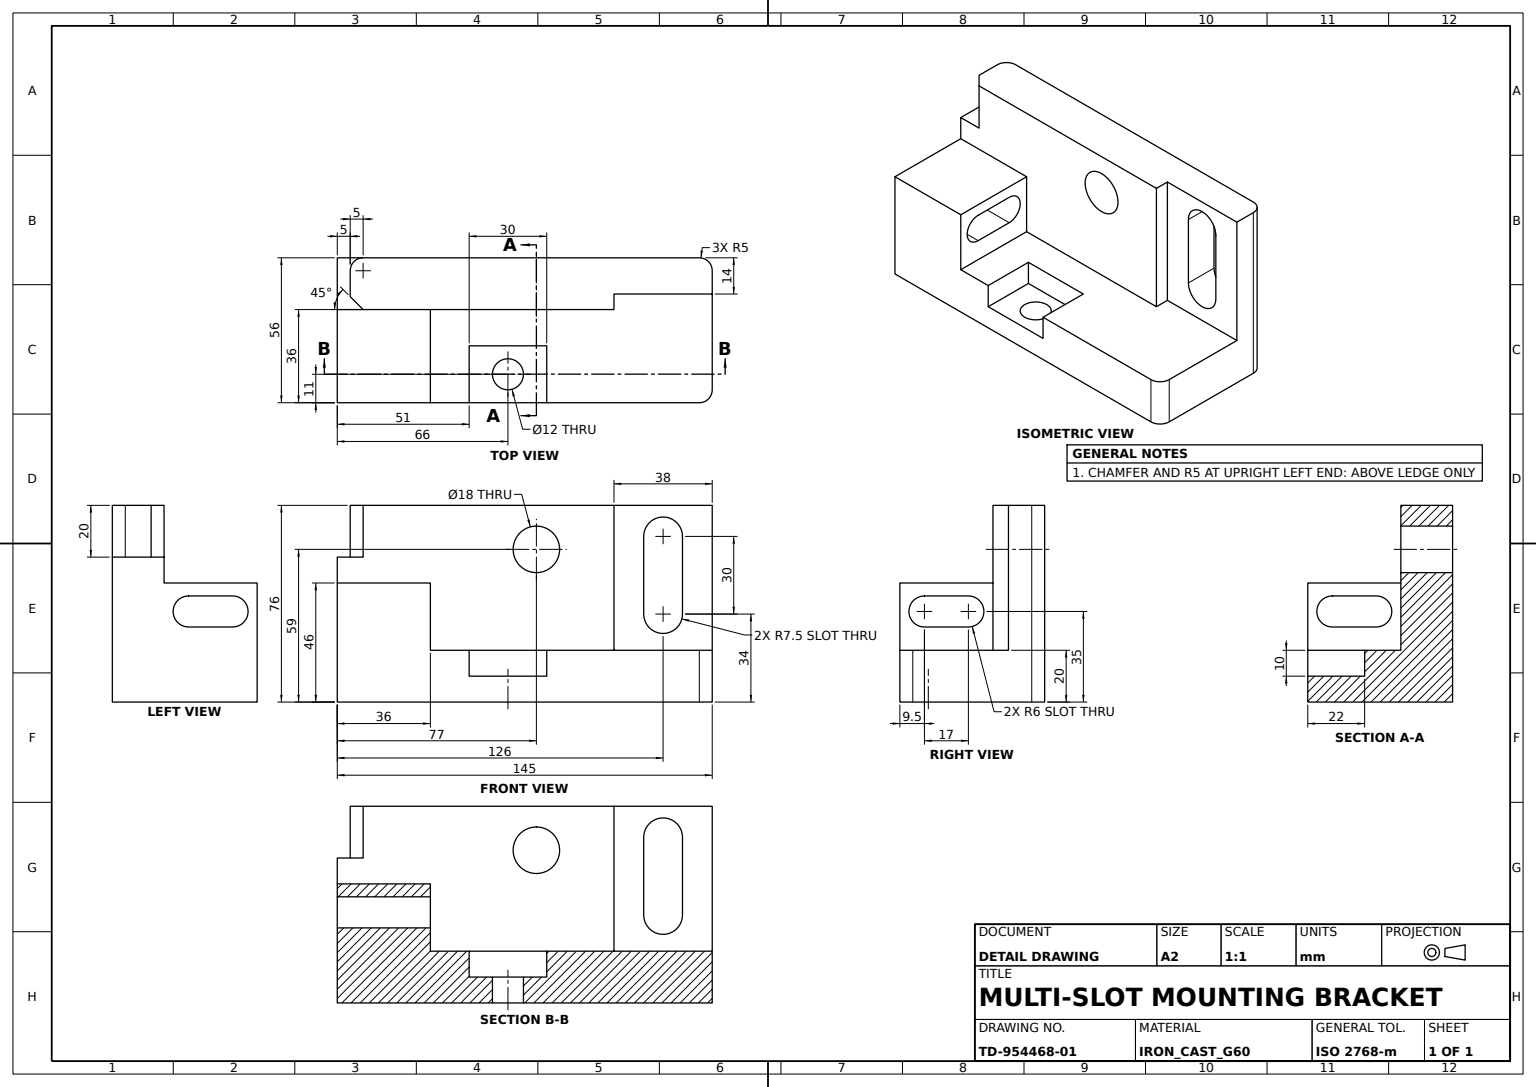
ISO-10303-21;
HEADER;
FILE_DESCRIPTION((''),'2;1');
FILE_NAME('','',(''),(''),'','','');
FILE_SCHEMA(('AUTOMOTIVE_DESIGN'));
ENDSEC;
DATA;
#1=APPLICATION_CONTEXT('');
#2=PRODUCT_CONTEXT('',#1,'mechanical');
#3=PRODUCT('','','',(#2));
#4=PRODUCT_DEFINITION_FORMATION('','',#3);
#5=PRODUCT_DEFINITION_CONTEXT('',#1,'design');
#6=PRODUCT_DEFINITION('','',#4,#5);
#7=PRODUCT_DEFINITION_SHAPE('','',#6);
#8=(LENGTH_UNIT()NAMED_UNIT(*)SI_UNIT(.MILLI.,.METRE.));
#9=(NAMED_UNIT(*)PLANE_ANGLE_UNIT()SI_UNIT($,.RADIAN.));
#10=(NAMED_UNIT(*)SI_UNIT($,.STERADIAN.)SOLID_ANGLE_UNIT());
#11=UNCERTAINTY_MEASURE_WITH_UNIT(LENGTH_MEASURE(0.005),#8,'distance_accuracy_value','');
#12=(GEOMETRIC_REPRESENTATION_CONTEXT(3)GLOBAL_UNCERTAINTY_ASSIGNED_CONTEXT((#11))GLOBAL_UNIT_ASSIGNED_CONTEXT((#8,#9,#10))REPRESENTATION_CONTEXT('',''));
#13=CARTESIAN_POINT('',(-12.5,-17.,10.));
#14=VERTEX_POINT('',#13);
#15=CARTESIAN_POINT('',(-6.5,-17.,10.));
#16=DIRECTION('',(0.,0.,-1.));
#17=DIRECTION('',(-1.,0.,0.));
#18=AXIS2_PLACEMENT_3D('',#15,#16,#17);
#19=CIRCLE('',#18,6.);
#20=EDGE_CURVE('',#14,#14,#19,.T.);
#21=ORIENTED_EDGE('',*,*,#20,.T.);
#22=EDGE_LOOP('',(#21));
#23=FACE_BOUND('',#22,.T.);
#24=CARTESIAN_POINT('',(-21.5,-6.,10.));
#25=VERTEX_POINT('',#24);
#26=CARTESIAN_POINT('',(-21.5,-28.,10.));
#27=VERTEX_POINT('',#26);
#28=CARTESIAN_POINT('',(-21.5,-40.,10.));
#29=DIRECTION('',(0.,1.,0.));
#30=VECTOR('',#29,1000.);
#31=LINE('',#28,#30);
#32=EDGE_CURVE('',#25,#27,#31,.F.);
#33=ORIENTED_EDGE('',*,*,#32,.T.);
#34=CARTESIAN_POINT('',(8.5,-28.,10.));
#35=VERTEX_POINT('',#34);
#36=CARTESIAN_POINT('',(72.5,-28.,10.));
#37=DIRECTION('',(1.,0.,0.));
#38=VECTOR('',#37,1000.);
#39=LINE('',#36,#38);
#40=EDGE_CURVE('',#27,#35,#39,.T.);
#41=ORIENTED_EDGE('',*,*,#40,.T.);
#42=CARTESIAN_POINT('',(8.5,-6.,10.));
#43=VERTEX_POINT('',#42);
#44=DIRECTION('',(0.,-1.,0.));
#45=VECTOR('',#44,1000.);
#46=LINE('',#42,#45);
#47=EDGE_CURVE('',#35,#43,#46,.F.);
#48=ORIENTED_EDGE('',*,*,#47,.T.);
#49=LINE('',#24,#38);
#50=EDGE_CURVE('',#43,#25,#49,.F.);
#51=ORIENTED_EDGE('',*,*,#50,.T.);
#52=EDGE_LOOP('',(#33,#41,#48,#51));
#53=FACE_BOUND('',#52,.T.);
#54=CARTESIAN_POINT('',(0.,0.,10.));
#55=AXIS2_PLACEMENT_3D('',#54,#16,#17);
#56=PLANE('',#55);
#57=ADVANCED_FACE('',(#23,#53),#56,.F.);
#58=CARTESIAN_POINT('',(-21.5,-28.,20.));
#59=VERTEX_POINT('',#58);
#60=CARTESIAN_POINT('',(-21.5,-6.,20.));
#61=VERTEX_POINT('',#60);
#62=CARTESIAN_POINT('',(-21.5,0.,20.));
#63=LINE('',#62,#30);
#64=EDGE_CURVE('',#59,#61,#63,.T.);
#65=ORIENTED_EDGE('',*,*,#64,.T.);
#66=CARTESIAN_POINT('',(8.5,-6.,20.));
#67=VERTEX_POINT('',#66);
#68=CARTESIAN_POINT('',(0.,-6.,20.));
#69=LINE('',#68,#38);
#70=EDGE_CURVE('',#61,#67,#69,.T.);
#71=ORIENTED_EDGE('',*,*,#70,.T.);
#72=CARTESIAN_POINT('',(8.5,-28.,20.));
#73=VERTEX_POINT('',#72);
#74=CARTESIAN_POINT('',(8.5,0.,20.));
#75=LINE('',#74,#45);
#76=EDGE_CURVE('',#67,#73,#75,.T.);
#77=ORIENTED_EDGE('',*,*,#76,.T.);
#78=CARTESIAN_POINT('',(67.5,-28.,20.));
#79=VERTEX_POINT('',#78);
#80=CARTESIAN_POINT('',(72.5,-28.,20.));
#81=VECTOR('',#17,1000.);
#82=LINE('',#80,#81);
#83=EDGE_CURVE('',#79,#73,#82,.T.);
#84=ORIENTED_EDGE('',*,*,#83,.F.);
#85=CARTESIAN_POINT('',(72.5,-23.,20.));
#86=VERTEX_POINT('',#85);
#87=CARTESIAN_POINT('',(67.5,-23.,20.));
#88=AXIS2_PLACEMENT_3D('',#87,#16,#17);
#89=CIRCLE('',#88,5.);
#90=EDGE_CURVE('',#79,#86,#89,.F.);
#91=ORIENTED_EDGE('',*,*,#90,.T.);
#92=CARTESIAN_POINT('',(72.5,14.,20.));
#93=VERTEX_POINT('',#92);
#94=CARTESIAN_POINT('',(72.5,28.,20.));
#95=LINE('',#94,#45);
#96=EDGE_CURVE('',#93,#86,#95,.T.);
#97=ORIENTED_EDGE('',*,*,#96,.F.);
#98=CARTESIAN_POINT('',(34.5,14.,20.));
#99=VERTEX_POINT('',#98);
#100=LINE('',#92,#81);
#101=EDGE_CURVE('',#99,#93,#100,.F.);
#102=ORIENTED_EDGE('',*,*,#101,.F.);
#103=CARTESIAN_POINT('',(34.5,8.,20.));
#104=VERTEX_POINT('',#103);
#105=LINE('',#98,#45);
#106=EDGE_CURVE('',#104,#99,#105,.F.);
#107=ORIENTED_EDGE('',*,*,#106,.F.);
#108=CARTESIAN_POINT('',(-36.5,8.,20.));
#109=VERTEX_POINT('',#108);
#110=CARTESIAN_POINT('',(0.,8.,20.));
#111=LINE('',#110,#81);
#112=EDGE_CURVE('',#104,#109,#111,.T.);
#113=ORIENTED_EDGE('',*,*,#112,.T.);
#114=CARTESIAN_POINT('',(-36.5,-28.,20.));
#115=VERTEX_POINT('',#114);
#116=CARTESIAN_POINT('',(-36.5,0.,20.));
#117=LINE('',#116,#45);
#118=EDGE_CURVE('',#109,#115,#117,.T.);
#119=ORIENTED_EDGE('',*,*,#118,.T.);
#120=EDGE_CURVE('',#59,#115,#82,.T.);
#121=ORIENTED_EDGE('',*,*,#120,.F.);
#122=EDGE_LOOP('',(#65,#71,#77,#84,#91,#97,#102,#107,#113,#119,#121));
#123=FACE_BOUND('',#122,.T.);
#124=CARTESIAN_POINT('',(0.,0.,20.));
#125=AXIS2_PLACEMENT_3D('',#124,#16,#17);
#126=PLANE('',#125);
#127=ADVANCED_FACE('',(#123),#126,.F.);
#128=CARTESIAN_POINT('',(-72.5,8.,56.));
#129=VERTEX_POINT('',#128);
#130=CARTESIAN_POINT('',(-62.5,8.,56.));
#131=VERTEX_POINT('',#130);
#132=CARTESIAN_POINT('',(72.5,8.,56.));
#133=LINE('',#132,#38);
#134=EDGE_CURVE('',#129,#131,#133,.T.);
#135=ORIENTED_EDGE('',*,*,#134,.T.);
#136=CARTESIAN_POINT('',(-67.5,13.,56.));
#137=VERTEX_POINT('',#136);
#138=CARTESIAN_POINT('',(-86.5,32.,56.));
#139=DIRECTION('',(-0.707106781,0.707106781,0.));
#140=VECTOR('',#139,1000.);
#141=LINE('',#138,#140);
#142=EDGE_CURVE('',#131,#137,#141,.T.);
#143=ORIENTED_EDGE('',*,*,#142,.T.);
#144=CARTESIAN_POINT('',(-67.5,23.,56.));
#145=VERTEX_POINT('',#144);
#146=CARTESIAN_POINT('',(-67.5,46.,56.));
#147=LINE('',#146,#45);
#148=EDGE_CURVE('',#137,#145,#147,.F.);
#149=ORIENTED_EDGE('',*,*,#148,.T.);
#150=CARTESIAN_POINT('',(-62.5,28.,56.));
#151=VERTEX_POINT('',#150);
#152=CARTESIAN_POINT('',(-62.5,23.,56.));
#153=AXIS2_PLACEMENT_3D('',#152,#16,#17);
#154=CIRCLE('',#153,5.);
#155=EDGE_CURVE('',#145,#151,#154,.T.);
#156=ORIENTED_EDGE('',*,*,#155,.T.);
#157=CARTESIAN_POINT('',(-72.5,28.,56.));
#158=VERTEX_POINT('',#157);
#159=LINE('',#157,#81);
#160=EDGE_CURVE('',#151,#158,#159,.T.);
#161=ORIENTED_EDGE('',*,*,#160,.T.);
#162=CARTESIAN_POINT('',(-72.5,46.,56.));
#163=LINE('',#162,#45);
#164=EDGE_CURVE('',#158,#129,#163,.T.);
#165=ORIENTED_EDGE('',*,*,#164,.T.);
#166=EDGE_LOOP('',(#135,#143,#149,#156,#161,#165));
#167=FACE_BOUND('',#166,.T.);
#168=AXIS2_PLACEMENT_3D('',#162,#16,#17);
#169=PLANE('',#168);
#170=ADVANCED_FACE('',(#167),#169,.F.);
#171=CARTESIAN_POINT('',(-72.5,8.,46.));
#172=VERTEX_POINT('',#171);
#173=CARTESIAN_POINT('',(-36.5,8.,46.));
#174=VERTEX_POINT('',#173);
#175=LINE('',#171,#38);
#176=EDGE_CURVE('',#172,#174,#175,.T.);
#177=ORIENTED_EDGE('',*,*,#176,.F.);
#178=CARTESIAN_POINT('',(-72.5,-28.,46.));
#179=VERTEX_POINT('',#178);
#180=LINE('',#178,#30);
#181=EDGE_CURVE('',#179,#172,#180,.T.);
#182=ORIENTED_EDGE('',*,*,#181,.F.);
#183=CARTESIAN_POINT('',(-36.5,-28.,46.));
#184=VERTEX_POINT('',#183);
#185=LINE('',#183,#81);
#186=EDGE_CURVE('',#184,#179,#185,.T.);
#187=ORIENTED_EDGE('',*,*,#186,.F.);
#188=LINE('',#173,#45);
#189=EDGE_CURVE('',#174,#184,#188,.T.);
#190=ORIENTED_EDGE('',*,*,#189,.F.);
#191=EDGE_LOOP('',(#177,#182,#187,#190));
#192=FACE_BOUND('',#191,.T.);
#193=CARTESIAN_POINT('',(0.,0.,46.));
#194=AXIS2_PLACEMENT_3D('',#193,#16,#17);
#195=PLANE('',#194);
#196=ADVANCED_FACE('',(#192),#195,.F.);
#197=CARTESIAN_POINT('',(46.,14.,34.));
#198=VERTEX_POINT('',#197);
#199=CARTESIAN_POINT('',(46.,14.,64.));
#200=VERTEX_POINT('',#199);
#201=CARTESIAN_POINT('',(46.,14.,87.5));
#202=DIRECTION('',(0.,0.,1.));
#203=VECTOR('',#202,1000.);
#204=LINE('',#201,#203);
#205=EDGE_CURVE('',#198,#200,#204,.T.);
#206=ORIENTED_EDGE('',*,*,#205,.T.);
#207=CARTESIAN_POINT('',(61.,14.,64.));
#208=VERTEX_POINT('',#207);
#209=CARTESIAN_POINT('',(53.5,14.,64.));
#210=AXIS2_PLACEMENT_3D('',#209,#44,#37);
#211=CIRCLE('',#210,7.5);
#212=EDGE_CURVE('',#200,#208,#211,.F.);
#213=ORIENTED_EDGE('',*,*,#212,.T.);
#214=CARTESIAN_POINT('',(61.,14.,34.));
#215=VERTEX_POINT('',#214);
#216=CARTESIAN_POINT('',(61.,14.,87.5));
#217=VECTOR('',#16,1000.);
#218=LINE('',#216,#217);
#219=EDGE_CURVE('',#208,#215,#218,.T.);
#220=ORIENTED_EDGE('',*,*,#219,.T.);
#221=CARTESIAN_POINT('',(53.5,14.,34.));
#222=AXIS2_PLACEMENT_3D('',#221,#44,#37);
#223=CIRCLE('',#222,7.5);
#224=EDGE_CURVE('',#215,#198,#223,.F.);
#225=ORIENTED_EDGE('',*,*,#224,.T.);
#226=EDGE_LOOP('',(#206,#213,#220,#225));
#227=FACE_BOUND('',#226,.T.);
#228=ORIENTED_EDGE('',*,*,#101,.T.);
#229=CARTESIAN_POINT('',(72.5,14.,76.));
#230=VERTEX_POINT('',#229);
#231=CARTESIAN_POINT('',(72.5,14.,87.5));
#232=LINE('',#231,#217);
#233=EDGE_CURVE('',#93,#230,#232,.F.);
#234=ORIENTED_EDGE('',*,*,#233,.T.);
#235=CARTESIAN_POINT('',(34.5,14.,76.));
#236=VERTEX_POINT('',#235);
#237=LINE('',#229,#38);
#238=EDGE_CURVE('',#236,#230,#237,.T.);
#239=ORIENTED_EDGE('',*,*,#238,.F.);
#240=CARTESIAN_POINT('',(34.5,14.,87.5));
#241=LINE('',#240,#217);
#242=EDGE_CURVE('',#236,#99,#241,.T.);
#243=ORIENTED_EDGE('',*,*,#242,.T.);
#244=EDGE_LOOP('',(#228,#234,#239,#243));
#245=FACE_BOUND('',#244,.T.);
#246=AXIS2_PLACEMENT_3D('',#231,#44,#37);
#247=PLANE('',#246);
#248=ADVANCED_FACE('',(#227,#245),#247,.T.);
#249=ORIENTED_EDGE('',*,*,#212,.F.);
#250=CARTESIAN_POINT('',(46.,28.,64.));
#251=VERTEX_POINT('',#250);
#252=CARTESIAN_POINT('',(46.,76.5,64.));
#253=LINE('',#252,#45);
#254=EDGE_CURVE('',#200,#251,#253,.F.);
#255=ORIENTED_EDGE('',*,*,#254,.T.);
#256=CARTESIAN_POINT('',(61.,28.,64.));
#257=VERTEX_POINT('',#256);
#258=CARTESIAN_POINT('',(53.5,28.,64.));
#259=AXIS2_PLACEMENT_3D('',#258,#29,#202);
#260=CIRCLE('',#259,7.5);
#261=EDGE_CURVE('',#257,#251,#260,.F.);
#262=ORIENTED_EDGE('',*,*,#261,.F.);
#263=CARTESIAN_POINT('',(61.,76.5,64.));
#264=LINE('',#263,#45);
#265=EDGE_CURVE('',#208,#257,#264,.F.);
#266=ORIENTED_EDGE('',*,*,#265,.F.);
#267=EDGE_LOOP('',(#249,#255,#262,#266));
#268=FACE_BOUND('',#267,.T.);
#269=CARTESIAN_POINT('',(53.5,76.5,64.));
#270=AXIS2_PLACEMENT_3D('',#269,#44,#16);
#271=CYLINDRICAL_SURFACE('',#270,7.5);
#272=ADVANCED_FACE('',(#268),#271,.F.);
#273=CARTESIAN_POINT('',(67.5,28.,76.));
#274=VERTEX_POINT('',#273);
#275=CARTESIAN_POINT('',(-62.5,28.,76.));
#276=VERTEX_POINT('',#275);
#277=CARTESIAN_POINT('',(72.5,28.,76.));
#278=LINE('',#277,#81);
#279=EDGE_CURVE('',#274,#276,#278,.T.);
#280=ORIENTED_EDGE('',*,*,#279,.T.);
#281=CARTESIAN_POINT('',(-67.5,23.,76.));
#282=VERTEX_POINT('',#281);
#283=CARTESIAN_POINT('',(-62.5,23.,76.));
#284=AXIS2_PLACEMENT_3D('',#283,#202,#37);
#285=CIRCLE('',#284,5.);
#286=EDGE_CURVE('',#276,#282,#285,.T.);
#287=ORIENTED_EDGE('',*,*,#286,.T.);
#288=CARTESIAN_POINT('',(-67.5,13.,76.));
#289=VERTEX_POINT('',#288);
#290=CARTESIAN_POINT('',(-67.5,8.,76.));
#291=LINE('',#290,#30);
#292=EDGE_CURVE('',#289,#282,#291,.T.);
#293=ORIENTED_EDGE('',*,*,#292,.F.);
#294=CARTESIAN_POINT('',(-62.5,8.,76.));
#295=VERTEX_POINT('',#294);
#296=CARTESIAN_POINT('',(5.,-59.5,76.));
#297=DIRECTION('',(0.707106781,-0.707106781,0.));
#298=VECTOR('',#297,1000.);
#299=LINE('',#296,#298);
#300=EDGE_CURVE('',#289,#295,#299,.T.);
#301=ORIENTED_EDGE('',*,*,#300,.T.);
#302=CARTESIAN_POINT('',(34.5,8.,76.));
#303=VERTEX_POINT('',#302);
#304=CARTESIAN_POINT('',(72.5,8.,76.));
#305=LINE('',#304,#81);
#306=EDGE_CURVE('',#303,#295,#305,.T.);
#307=ORIENTED_EDGE('',*,*,#306,.F.);
#308=LINE('',#302,#30);
#309=EDGE_CURVE('',#236,#303,#308,.F.);
#310=ORIENTED_EDGE('',*,*,#309,.F.);
#311=ORIENTED_EDGE('',*,*,#238,.T.);
#312=CARTESIAN_POINT('',(72.5,23.,76.));
#313=VERTEX_POINT('',#312);
#314=LINE('',#304,#30);
#315=EDGE_CURVE('',#230,#313,#314,.T.);
#316=ORIENTED_EDGE('',*,*,#315,.T.);
#317=CARTESIAN_POINT('',(67.5,23.,76.));
#318=AXIS2_PLACEMENT_3D('',#317,#202,#37);
#319=CIRCLE('',#318,5.);
#320=EDGE_CURVE('',#313,#274,#319,.T.);
#321=ORIENTED_EDGE('',*,*,#320,.T.);
#322=EDGE_LOOP('',(#280,#287,#293,#301,#307,#310,#311,#316,#321));
#323=FACE_BOUND('',#322,.T.);
#324=AXIS2_PLACEMENT_3D('',#304,#202,#37);
#325=PLANE('',#324);
#326=ADVANCED_FACE('',(#323),#325,.T.);
#327=ORIENTED_EDGE('',*,*,#205,.F.);
#328=CARTESIAN_POINT('',(46.,28.,34.));
#329=VERTEX_POINT('',#328);
#330=CARTESIAN_POINT('',(46.,76.5,34.));
#331=LINE('',#330,#45);
#332=EDGE_CURVE('',#198,#329,#331,.F.);
#333=ORIENTED_EDGE('',*,*,#332,.T.);
#334=CARTESIAN_POINT('',(46.,28.,20.));
#335=LINE('',#334,#217);
#336=EDGE_CURVE('',#251,#329,#335,.T.);
#337=ORIENTED_EDGE('',*,*,#336,.F.);
#338=ORIENTED_EDGE('',*,*,#254,.F.);
#339=EDGE_LOOP('',(#327,#333,#337,#338));
#340=FACE_BOUND('',#339,.T.);
#341=AXIS2_PLACEMENT_3D('',#330,#37,#16);
#342=PLANE('',#341);
#343=ADVANCED_FACE('',(#340),#342,.T.);
#344=ORIENTED_EDGE('',*,*,#155,.F.);
#345=LINE('',#144,#203);
#346=EDGE_CURVE('',#282,#145,#345,.F.);
#347=ORIENTED_EDGE('',*,*,#346,.F.);
#348=ORIENTED_EDGE('',*,*,#286,.F.);
#349=LINE('',#275,#203);
#350=EDGE_CURVE('',#151,#276,#349,.T.);
#351=ORIENTED_EDGE('',*,*,#350,.F.);
#352=EDGE_LOOP('',(#344,#347,#348,#351));
#353=FACE_BOUND('',#352,.T.);
#354=CARTESIAN_POINT('',(-62.5,23.,20.));
#355=AXIS2_PLACEMENT_3D('',#354,#16,#17);
#356=CYLINDRICAL_SURFACE('',#355,5.);
#357=ADVANCED_FACE('',(#353),#356,.T.);
#358=CARTESIAN_POINT('',(-72.5,28.,0.));
#359=VERTEX_POINT('',#358);
#360=CARTESIAN_POINT('',(-72.5,28.,20.));
#361=LINE('',#360,#217);
#362=EDGE_CURVE('',#158,#359,#361,.T.);
#363=ORIENTED_EDGE('',*,*,#362,.T.);
#364=CARTESIAN_POINT('',(-72.5,-28.,0.));
#365=VERTEX_POINT('',#364);
#366=LINE('',#364,#30);
#367=EDGE_CURVE('',#365,#359,#366,.T.);
#368=ORIENTED_EDGE('',*,*,#367,.F.);
#369=CARTESIAN_POINT('',(-72.5,-28.,20.));
#370=LINE('',#369,#217);
#371=EDGE_CURVE('',#179,#365,#370,.T.);
#372=ORIENTED_EDGE('',*,*,#371,.F.);
#373=ORIENTED_EDGE('',*,*,#181,.T.);
#374=CARTESIAN_POINT('',(-72.5,8.,0.));
#375=LINE('',#374,#203);
#376=EDGE_CURVE('',#172,#129,#375,.T.);
#377=ORIENTED_EDGE('',*,*,#376,.T.);
#378=ORIENTED_EDGE('',*,*,#164,.F.);
#379=EDGE_LOOP('',(#363,#368,#372,#373,#377,#378));
#380=FACE_BOUND('',#379,.T.);
#381=CARTESIAN_POINT('',(-72.5,-18.5,41.));
#382=VERTEX_POINT('',#381);
#383=CARTESIAN_POINT('',(-72.5,-18.5,29.));
#384=VERTEX_POINT('',#383);
#385=CARTESIAN_POINT('',(-72.5,-18.5,35.));
#386=AXIS2_PLACEMENT_3D('',#385,#17,#202);
#387=CIRCLE('',#386,6.);
#388=EDGE_CURVE('',#382,#384,#387,.F.);
#389=ORIENTED_EDGE('',*,*,#388,.T.);
#390=CARTESIAN_POINT('',(-72.5,-1.5,29.));
#391=VERTEX_POINT('',#390);
#392=CARTESIAN_POINT('',(-72.5,-28.,29.));
#393=LINE('',#392,#30);
#394=EDGE_CURVE('',#384,#391,#393,.T.);
#395=ORIENTED_EDGE('',*,*,#394,.T.);
#396=CARTESIAN_POINT('',(-72.5,-1.5,41.));
#397=VERTEX_POINT('',#396);
#398=CARTESIAN_POINT('',(-72.5,-1.5,35.));
#399=AXIS2_PLACEMENT_3D('',#398,#17,#202);
#400=CIRCLE('',#399,6.);
#401=EDGE_CURVE('',#391,#397,#400,.F.);
#402=ORIENTED_EDGE('',*,*,#401,.T.);
#403=CARTESIAN_POINT('',(-72.5,-28.,41.));
#404=LINE('',#403,#45);
#405=EDGE_CURVE('',#397,#382,#404,.T.);
#406=ORIENTED_EDGE('',*,*,#405,.T.);
#407=EDGE_LOOP('',(#389,#395,#402,#406));
#408=FACE_BOUND('',#407,.T.);
#409=AXIS2_PLACEMENT_3D('',#369,#17,#202);
#410=PLANE('',#409);
#411=ADVANCED_FACE('',(#380,#408),#410,.T.);
#412=LINE('',#130,#217);
#413=EDGE_CURVE('',#295,#131,#412,.T.);
#414=ORIENTED_EDGE('',*,*,#413,.F.);
#415=ORIENTED_EDGE('',*,*,#300,.F.);
#416=LINE('',#288,#203);
#417=EDGE_CURVE('',#137,#289,#416,.T.);
#418=ORIENTED_EDGE('',*,*,#417,.F.);
#419=ORIENTED_EDGE('',*,*,#142,.F.);
#420=EDGE_LOOP('',(#414,#415,#418,#419));
#421=FACE_BOUND('',#420,.T.);
#422=DIRECTION('',(-0.707106781,-0.707106781,0.));
#423=AXIS2_PLACEMENT_3D('',#136,#422,#16);
#424=PLANE('',#423);
#425=ADVANCED_FACE('',(#421),#424,.T.);
#426=CARTESIAN_POINT('',(67.5,28.,0.));
#427=VERTEX_POINT('',#426);
#428=CARTESIAN_POINT('',(72.5,23.,0.));
#429=VERTEX_POINT('',#428);
#430=CARTESIAN_POINT('',(67.5,23.,0.));
#431=AXIS2_PLACEMENT_3D('',#430,#16,#17);
#432=CIRCLE('',#431,5.);
#433=EDGE_CURVE('',#427,#429,#432,.T.);
#434=ORIENTED_EDGE('',*,*,#433,.T.);
#435=CARTESIAN_POINT('',(72.5,-23.,0.));
#436=VERTEX_POINT('',#435);
#437=CARTESIAN_POINT('',(72.5,28.,0.));
#438=LINE('',#437,#45);
#439=EDGE_CURVE('',#429,#436,#438,.T.);
#440=ORIENTED_EDGE('',*,*,#439,.T.);
#441=CARTESIAN_POINT('',(67.5,-28.,0.));
#442=VERTEX_POINT('',#441);
#443=CARTESIAN_POINT('',(67.5,-23.,0.));
#444=AXIS2_PLACEMENT_3D('',#443,#16,#17);
#445=CIRCLE('',#444,5.);
#446=EDGE_CURVE('',#436,#442,#445,.T.);
#447=ORIENTED_EDGE('',*,*,#446,.T.);
#448=CARTESIAN_POINT('',(72.5,-28.,0.));
#449=LINE('',#448,#81);
#450=EDGE_CURVE('',#442,#365,#449,.T.);
#451=ORIENTED_EDGE('',*,*,#450,.T.);
#452=ORIENTED_EDGE('',*,*,#367,.T.);
#453=LINE('',#358,#38);
#454=EDGE_CURVE('',#359,#427,#453,.T.);
#455=ORIENTED_EDGE('',*,*,#454,.T.);
#456=EDGE_LOOP('',(#434,#440,#447,#451,#452,#455));
#457=FACE_BOUND('',#456,.T.);
#458=CARTESIAN_POINT('',(-12.5,-17.,0.));
#459=VERTEX_POINT('',#458);
#460=CARTESIAN_POINT('',(-6.5,-17.,0.));
#461=AXIS2_PLACEMENT_3D('',#460,#16,#17);
#462=CIRCLE('',#461,6.);
#463=EDGE_CURVE('',#459,#459,#462,.T.);
#464=ORIENTED_EDGE('',*,*,#463,.F.);
#465=EDGE_LOOP('',(#464));
#466=FACE_BOUND('',#465,.T.);
#467=CARTESIAN_POINT('',(0.,0.,0.));
#468=AXIS2_PLACEMENT_3D('',#467,#16,#17);
#469=PLANE('',#468);
#470=ADVANCED_FACE('',(#457,#466),#469,.T.);
#471=CARTESIAN_POINT('',(-36.5,-18.5,29.));
#472=VERTEX_POINT('',#471);
#473=CARTESIAN_POINT('',(-76.5,-18.5,29.));
#474=LINE('',#473,#38);
#475=EDGE_CURVE('',#472,#384,#474,.F.);
#476=ORIENTED_EDGE('',*,*,#475,.F.);
#477=CARTESIAN_POINT('',(-36.5,-1.5,29.));
#478=VERTEX_POINT('',#477);
#479=CARTESIAN_POINT('',(-36.5,8.,29.));
#480=LINE('',#479,#45);
#481=EDGE_CURVE('',#478,#472,#480,.T.);
#482=ORIENTED_EDGE('',*,*,#481,.F.);
#483=CARTESIAN_POINT('',(-76.5,-1.5,29.));
#484=LINE('',#483,#38);
#485=EDGE_CURVE('',#478,#391,#484,.F.);
#486=ORIENTED_EDGE('',*,*,#485,.T.);
#487=ORIENTED_EDGE('',*,*,#394,.F.);
#488=EDGE_LOOP('',(#476,#482,#486,#487));
#489=FACE_BOUND('',#488,.T.);
#490=AXIS2_PLACEMENT_3D('',#483,#202,#37);
#491=PLANE('',#490);
#492=ADVANCED_FACE('',(#489),#491,.T.);
#493=ORIENTED_EDGE('',*,*,#475,.T.);
#494=ORIENTED_EDGE('',*,*,#388,.F.);
#495=CARTESIAN_POINT('',(-36.5,-18.5,41.));
#496=VERTEX_POINT('',#495);
#497=CARTESIAN_POINT('',(-76.5,-18.5,41.));
#498=LINE('',#497,#38);
#499=EDGE_CURVE('',#496,#382,#498,.F.);
#500=ORIENTED_EDGE('',*,*,#499,.F.);
#501=CARTESIAN_POINT('',(-36.5,-18.5,35.));
#502=AXIS2_PLACEMENT_3D('',#501,#37,#29);
#503=CIRCLE('',#502,6.);
#504=EDGE_CURVE('',#472,#496,#503,.F.);
#505=ORIENTED_EDGE('',*,*,#504,.F.);
#506=EDGE_LOOP('',(#493,#494,#500,#505));
#507=FACE_BOUND('',#506,.T.);
#508=CARTESIAN_POINT('',(-76.5,-18.5,35.));
#509=AXIS2_PLACEMENT_3D('',#508,#37,#16);
#510=CYLINDRICAL_SURFACE('',#509,6.);
#511=ADVANCED_FACE('',(#507),#510,.F.);
#512=ORIENTED_EDGE('',*,*,#481,.T.);
#513=ORIENTED_EDGE('',*,*,#504,.T.);
#514=CARTESIAN_POINT('',(-36.5,-1.5,41.));
#515=VERTEX_POINT('',#514);
#516=CARTESIAN_POINT('',(-36.5,8.,41.));
#517=LINE('',#516,#30);
#518=EDGE_CURVE('',#496,#515,#517,.T.);
#519=ORIENTED_EDGE('',*,*,#518,.T.);
#520=CARTESIAN_POINT('',(-36.5,-1.5,35.));
#521=AXIS2_PLACEMENT_3D('',#520,#37,#29);
#522=CIRCLE('',#521,6.);
#523=EDGE_CURVE('',#515,#478,#522,.F.);
#524=ORIENTED_EDGE('',*,*,#523,.T.);
#525=EDGE_LOOP('',(#512,#513,#519,#524));
#526=FACE_BOUND('',#525,.T.);
#527=ORIENTED_EDGE('',*,*,#189,.T.);
#528=LINE('',#183,#217);
#529=EDGE_CURVE('',#184,#115,#528,.T.);
#530=ORIENTED_EDGE('',*,*,#529,.T.);
#531=ORIENTED_EDGE('',*,*,#118,.F.);
#532=LINE('',#173,#217);
#533=EDGE_CURVE('',#174,#109,#532,.T.);
#534=ORIENTED_EDGE('',*,*,#533,.F.);
#535=EDGE_LOOP('',(#527,#530,#531,#534));
#536=FACE_BOUND('',#535,.T.);
#537=AXIS2_PLACEMENT_3D('',#173,#37,#29);
#538=PLANE('',#537);
#539=ADVANCED_FACE('',(#526,#536),#538,.T.);
#540=ORIENTED_EDGE('',*,*,#463,.T.);
#541=EDGE_LOOP('',(#540));
#542=FACE_BOUND('',#541,.T.);
#543=ORIENTED_EDGE('',*,*,#20,.F.);
#544=EDGE_LOOP('',(#543));
#545=FACE_BOUND('',#544,.T.);
#546=CYLINDRICAL_SURFACE('',#18,6.);
#547=ADVANCED_FACE('',(#542,#545),#546,.F.);
#548=LINE('',#58,#217);
#549=EDGE_CURVE('',#59,#27,#548,.T.);
#550=ORIENTED_EDGE('',*,*,#549,.F.);
#551=ORIENTED_EDGE('',*,*,#120,.T.);
#552=ORIENTED_EDGE('',*,*,#529,.F.);
#553=ORIENTED_EDGE('',*,*,#186,.T.);
#554=ORIENTED_EDGE('',*,*,#371,.T.);
#555=ORIENTED_EDGE('',*,*,#450,.F.);
#556=LINE('',#78,#217);
#557=EDGE_CURVE('',#442,#79,#556,.F.);
#558=ORIENTED_EDGE('',*,*,#557,.T.);
#559=ORIENTED_EDGE('',*,*,#83,.T.);
#560=LINE('',#72,#203);
#561=EDGE_CURVE('',#35,#73,#560,.T.);
#562=ORIENTED_EDGE('',*,*,#561,.F.);
#563=ORIENTED_EDGE('',*,*,#40,.F.);
#564=EDGE_LOOP('',(#550,#551,#552,#553,#554,#555,#558,#559,#562,#563));
#565=FACE_BOUND('',#564,.T.);
#566=AXIS2_PLACEMENT_3D('',#80,#44,#16);
#567=PLANE('',#566);
#568=ADVANCED_FACE('',(#565),#567,.T.);
#569=ORIENTED_EDGE('',*,*,#499,.T.);
#570=ORIENTED_EDGE('',*,*,#405,.F.);
#571=CARTESIAN_POINT('',(-76.5,-1.5,41.));
#572=LINE('',#571,#38);
#573=EDGE_CURVE('',#515,#397,#572,.F.);
#574=ORIENTED_EDGE('',*,*,#573,.F.);
#575=ORIENTED_EDGE('',*,*,#518,.F.);
#576=EDGE_LOOP('',(#569,#570,#574,#575));
#577=FACE_BOUND('',#576,.T.);
#578=AXIS2_PLACEMENT_3D('',#497,#16,#17);
#579=PLANE('',#578);
#580=ADVANCED_FACE('',(#577),#579,.T.);
#581=ORIENTED_EDGE('',*,*,#32,.F.);
#582=CARTESIAN_POINT('',(-21.5,-6.,35.));
#583=LINE('',#582,#217);
#584=EDGE_CURVE('',#25,#61,#583,.F.);
#585=ORIENTED_EDGE('',*,*,#584,.T.);
#586=ORIENTED_EDGE('',*,*,#64,.F.);
#587=ORIENTED_EDGE('',*,*,#549,.T.);
#588=EDGE_LOOP('',(#581,#585,#586,#587));
#589=FACE_BOUND('',#588,.T.);
#590=CARTESIAN_POINT('',(-21.5,-40.,35.));
#591=AXIS2_PLACEMENT_3D('',#590,#17,#44);
#592=PLANE('',#591);
#593=ADVANCED_FACE('',(#589),#592,.F.);
#594=ORIENTED_EDGE('',*,*,#47,.F.);
#595=ORIENTED_EDGE('',*,*,#561,.T.);
#596=ORIENTED_EDGE('',*,*,#76,.F.);
#597=CARTESIAN_POINT('',(8.5,-6.,35.));
#598=LINE('',#597,#217);
#599=EDGE_CURVE('',#43,#67,#598,.F.);
#600=ORIENTED_EDGE('',*,*,#599,.F.);
#601=EDGE_LOOP('',(#594,#595,#596,#600));
#602=FACE_BOUND('',#601,.T.);
#603=AXIS2_PLACEMENT_3D('',#597,#37,#29);
#604=PLANE('',#603);
#605=ADVANCED_FACE('',(#602),#604,.F.);
#606=CARTESIAN_POINT('',(4.5,28.,68.));
#607=VERTEX_POINT('',#606);
#608=CARTESIAN_POINT('',(4.5,28.,59.));
#609=AXIS2_PLACEMENT_3D('',#608,#29,#202);
#610=CIRCLE('',#609,9.);
#611=EDGE_CURVE('',#607,#607,#610,.T.);
#612=ORIENTED_EDGE('',*,*,#611,.F.);
#613=EDGE_LOOP('',(#612));
#614=FACE_BOUND('',#613,.T.);
#615=CARTESIAN_POINT('',(61.,28.,34.));
#616=VERTEX_POINT('',#615);
#617=CARTESIAN_POINT('',(61.,28.,20.));
#618=LINE('',#617,#203);
#619=EDGE_CURVE('',#616,#257,#618,.T.);
#620=ORIENTED_EDGE('',*,*,#619,.T.);
#621=ORIENTED_EDGE('',*,*,#261,.T.);
#622=ORIENTED_EDGE('',*,*,#336,.T.);
#623=CARTESIAN_POINT('',(53.5,28.,34.));
#624=AXIS2_PLACEMENT_3D('',#623,#29,#202);
#625=CIRCLE('',#624,7.5);
#626=EDGE_CURVE('',#329,#616,#625,.F.);
#627=ORIENTED_EDGE('',*,*,#626,.T.);
#628=EDGE_LOOP('',(#620,#621,#622,#627));
#629=FACE_BOUND('',#628,.T.);
#630=CARTESIAN_POINT('',(67.5,28.,20.));
#631=LINE('',#630,#217);
#632=EDGE_CURVE('',#274,#427,#631,.T.);
#633=ORIENTED_EDGE('',*,*,#632,.T.);
#634=ORIENTED_EDGE('',*,*,#454,.F.);
#635=ORIENTED_EDGE('',*,*,#362,.F.);
#636=ORIENTED_EDGE('',*,*,#160,.F.);
#637=ORIENTED_EDGE('',*,*,#350,.T.);
#638=ORIENTED_EDGE('',*,*,#279,.F.);
#639=EDGE_LOOP('',(#633,#634,#635,#636,#637,#638));
#640=FACE_BOUND('',#639,.T.);
#641=AXIS2_PLACEMENT_3D('',#360,#29,#202);
#642=PLANE('',#641);
#643=ADVANCED_FACE('',(#614,#629,#640),#642,.T.);
#644=ORIENTED_EDGE('',*,*,#265,.T.);
#645=ORIENTED_EDGE('',*,*,#619,.F.);
#646=CARTESIAN_POINT('',(61.,76.5,34.));
#647=LINE('',#646,#45);
#648=EDGE_CURVE('',#215,#616,#647,.F.);
#649=ORIENTED_EDGE('',*,*,#648,.F.);
#650=ORIENTED_EDGE('',*,*,#219,.F.);
#651=EDGE_LOOP('',(#644,#645,#649,#650));
#652=FACE_BOUND('',#651,.T.);
#653=AXIS2_PLACEMENT_3D('',#263,#17,#202);
#654=PLANE('',#653);
#655=ADVANCED_FACE('',(#652),#654,.T.);
#656=LINE('',#85,#217);
#657=EDGE_CURVE('',#86,#436,#656,.T.);
#658=ORIENTED_EDGE('',*,*,#657,.T.);
#659=ORIENTED_EDGE('',*,*,#439,.F.);
#660=CARTESIAN_POINT('',(72.5,23.,20.));
#661=LINE('',#660,#217);
#662=EDGE_CURVE('',#429,#313,#661,.F.);
#663=ORIENTED_EDGE('',*,*,#662,.T.);
#664=ORIENTED_EDGE('',*,*,#315,.F.);
#665=ORIENTED_EDGE('',*,*,#233,.F.);
#666=ORIENTED_EDGE('',*,*,#96,.T.);
#667=EDGE_LOOP('',(#658,#659,#663,#664,#665,#666));
#668=FACE_BOUND('',#667,.T.);
#669=AXIS2_PLACEMENT_3D('',#94,#37,#16);
#670=PLANE('',#669);
#671=ADVANCED_FACE('',(#668),#670,.T.);
#672=ORIENTED_EDGE('',*,*,#320,.F.);
#673=ORIENTED_EDGE('',*,*,#662,.F.);
#674=ORIENTED_EDGE('',*,*,#433,.F.);
#675=ORIENTED_EDGE('',*,*,#632,.F.);
#676=EDGE_LOOP('',(#672,#673,#674,#675));
#677=FACE_BOUND('',#676,.T.);
#678=CARTESIAN_POINT('',(67.5,23.,20.));
#679=AXIS2_PLACEMENT_3D('',#678,#16,#17);
#680=CYLINDRICAL_SURFACE('',#679,5.);
#681=ADVANCED_FACE('',(#677),#680,.T.);
#682=ORIENTED_EDGE('',*,*,#292,.T.);
#683=ORIENTED_EDGE('',*,*,#346,.T.);
#684=ORIENTED_EDGE('',*,*,#148,.F.);
#685=ORIENTED_EDGE('',*,*,#417,.T.);
#686=EDGE_LOOP('',(#682,#683,#684,#685));
#687=FACE_BOUND('',#686,.T.);
#688=AXIS2_PLACEMENT_3D('',#146,#37,#16);
#689=PLANE('',#688);
#690=ADVANCED_FACE('',(#687),#689,.F.);
#691=ORIENTED_EDGE('',*,*,#70,.F.);
#692=ORIENTED_EDGE('',*,*,#584,.F.);
#693=ORIENTED_EDGE('',*,*,#50,.F.);
#694=ORIENTED_EDGE('',*,*,#599,.T.);
#695=EDGE_LOOP('',(#691,#692,#693,#694));
#696=FACE_BOUND('',#695,.T.);
#697=AXIS2_PLACEMENT_3D('',#582,#29,#202);
#698=PLANE('',#697);
#699=ADVANCED_FACE('',(#696),#698,.F.);
#700=CARTESIAN_POINT('',(4.5,8.,68.));
#701=VERTEX_POINT('',#700);
#702=CARTESIAN_POINT('',(4.5,8.,59.));
#703=AXIS2_PLACEMENT_3D('',#702,#29,#202);
#704=CIRCLE('',#703,9.);
#705=EDGE_CURVE('',#701,#701,#704,.T.);
#706=ORIENTED_EDGE('',*,*,#705,.F.);
#707=EDGE_LOOP('',(#706));
#708=FACE_BOUND('',#707,.T.);
#709=ORIENTED_EDGE('',*,*,#611,.T.);
#710=EDGE_LOOP('',(#709));
#711=FACE_BOUND('',#710,.T.);
#712=CYLINDRICAL_SURFACE('',#703,9.);
#713=ADVANCED_FACE('',(#708,#711),#712,.F.);
#714=ORIENTED_EDGE('',*,*,#401,.F.);
#715=ORIENTED_EDGE('',*,*,#485,.F.);
#716=ORIENTED_EDGE('',*,*,#523,.F.);
#717=ORIENTED_EDGE('',*,*,#573,.T.);
#718=EDGE_LOOP('',(#714,#715,#716,#717));
#719=FACE_BOUND('',#718,.T.);
#720=CARTESIAN_POINT('',(-76.5,-1.5,35.));
#721=AXIS2_PLACEMENT_3D('',#720,#37,#16);
#722=CYLINDRICAL_SURFACE('',#721,6.);
#723=ADVANCED_FACE('',(#719),#722,.F.);
#724=ORIENTED_EDGE('',*,*,#705,.T.);
#725=EDGE_LOOP('',(#724));
#726=FACE_BOUND('',#725,.T.);
#727=ORIENTED_EDGE('',*,*,#376,.F.);
#728=ORIENTED_EDGE('',*,*,#176,.T.);
#729=ORIENTED_EDGE('',*,*,#533,.T.);
#730=ORIENTED_EDGE('',*,*,#112,.F.);
#731=CARTESIAN_POINT('',(34.5,8.,87.5));
#732=LINE('',#731,#217);
#733=EDGE_CURVE('',#303,#104,#732,.T.);
#734=ORIENTED_EDGE('',*,*,#733,.F.);
#735=ORIENTED_EDGE('',*,*,#306,.T.);
#736=ORIENTED_EDGE('',*,*,#413,.T.);
#737=ORIENTED_EDGE('',*,*,#134,.F.);
#738=EDGE_LOOP('',(#727,#728,#729,#730,#734,#735,#736,#737));
#739=FACE_BOUND('',#738,.T.);
#740=CARTESIAN_POINT('',(72.5,8.,0.));
#741=AXIS2_PLACEMENT_3D('',#740,#44,#16);
#742=PLANE('',#741);
#743=ADVANCED_FACE('',(#726,#739),#742,.T.);
#744=ORIENTED_EDGE('',*,*,#648,.T.);
#745=ORIENTED_EDGE('',*,*,#626,.F.);
#746=ORIENTED_EDGE('',*,*,#332,.F.);
#747=ORIENTED_EDGE('',*,*,#224,.F.);
#748=EDGE_LOOP('',(#744,#745,#746,#747));
#749=FACE_BOUND('',#748,.T.);
#750=CARTESIAN_POINT('',(53.5,76.5,34.));
#751=AXIS2_PLACEMENT_3D('',#750,#44,#16);
#752=CYLINDRICAL_SURFACE('',#751,7.5);
#753=ADVANCED_FACE('',(#749),#752,.F.);
#754=ORIENTED_EDGE('',*,*,#309,.T.);
#755=ORIENTED_EDGE('',*,*,#733,.T.);
#756=ORIENTED_EDGE('',*,*,#106,.T.);
#757=ORIENTED_EDGE('',*,*,#242,.F.);
#758=EDGE_LOOP('',(#754,#755,#756,#757));
#759=FACE_BOUND('',#758,.T.);
#760=AXIS2_PLACEMENT_3D('',#240,#37,#16);
#761=PLANE('',#760);
#762=ADVANCED_FACE('',(#759),#761,.T.);
#763=ORIENTED_EDGE('',*,*,#657,.F.);
#764=ORIENTED_EDGE('',*,*,#90,.F.);
#765=ORIENTED_EDGE('',*,*,#557,.F.);
#766=ORIENTED_EDGE('',*,*,#446,.F.);
#767=EDGE_LOOP('',(#763,#764,#765,#766));
#768=FACE_BOUND('',#767,.T.);
#769=CYLINDRICAL_SURFACE('',#88,5.);
#770=ADVANCED_FACE('',(#768),#769,.T.);
#771=CLOSED_SHELL('',(#57,#127,#170,#196,#248,#272,#326,#343,#357,#411,#425,#470,#492,#511,#539,#547,#568,#580,#593,#605,#643,#655,#671,#681,#690,#699,#713,#723,#743,#753,#762,#770));
#772=MANIFOLD_SOLID_BREP('',#771);
#773=ADVANCED_BREP_SHAPE_REPRESENTATION('',(#772),#12);
#774=SHAPE_DEFINITION_REPRESENTATION(#7,#773);
ENDSEC;
END-ISO-10303-21;
